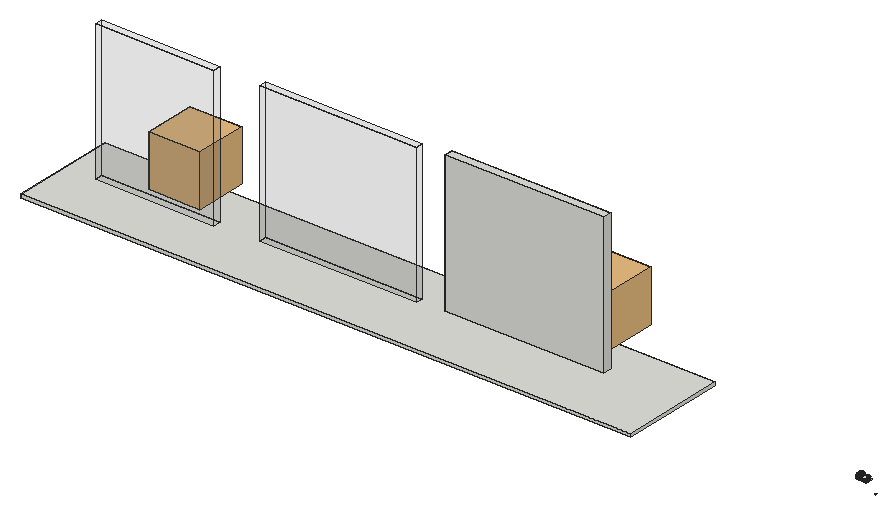
# SketchUp Ruby script. Lengths in inches.
U = 1.inch
M = Sketchup.active_model
def pt(a) = Geom::Point3d.new(a.map { |v| v * U })
def face(e, loops, mat)
  f = e.add_face(loops[0].map { |a| pt(a) })
  loops[1..].each { |l| e.add_face(l.map { |a| pt(a) }).erase! }
  f.material = f.back_material = mat if mat
  f
end
# faces: each face lists its corners as indices into pts; further lists are holes
def faces(e, pts, list, mat = nil) = list.each { |f| face(e, (f[0].is_a?(Array) ? f : [f]).map { |l| l.map { |i| pts[i] } }, mat) }
# xy, xz, yz: faces in a plane at the given z, y or x. An outline is a flat list of corners, or four numbers for a rectangle; further outlines are holes
def ring(l) = l.size == 4 ? [[l[0], l[1]], [l[2], l[1]], [l[2], l[3]], [l[0], l[3]]] : l.each_slice(2).to_a
def flat(e, list, mat, &to3) = list.each { |f| face(e, (f[0].is_a?(Array) ? f : [f]).map { |l| ring(l).map { |u, v| to3.(u, v) } }, mat) }
def xy(e, z, list, mat = nil) = flat(e, list, mat) { |x, y| [x, y, z] }
def xz(e, y, list, mat = nil) = flat(e, list, mat) { |x, z| [x, y, z] }
def yz(e, x, list, mat = nil) = flat(e, list, mat) { |y, z| [x, y, z] }
def lines(e, pts, list) = list.each { |a, b| e.add_line(pt(pts[a]), pt(pts[b])) }
# prism: a flat outline (further loops are holes) pulled along v
def prism(e, loops, v, mat = nil)
  f = face(e, loops, mat); d = Geom::Vector3d.new(v.map { |x| x * U })
  f.pushpull(f.normal.samedirection?(d) ? d.length : -d.length)
end
def box(e, o, s, mat = nil) = prism(e, [[o, [o[0] + s[0], o[1], o[2]], [o[0] + s[0], o[1] + s[1], o[2]], [o[0], o[1] + s[1], o[2]]]], [0, 0, s[2]], mat)
def at(x, y, z, deg = 0) = Geom::Transformation.translation(pt([x, y, z])) * Geom::Transformation.rotation(ORIGIN, Z_AXIS, deg.degrees)
def axes(o, x, y, z) = Geom::Transformation.new([*x, 0, *y, 0, *z, 0, *pt(o).to_a, 1])
def part(name) = M.definitions.add(name)
# library, detail: a bought-in or finely detailed component or shape, given as its bounding box
def library(name, o, s) = part(name).tap { |d| box(d.entities, o, s) }
def detail(e, o, s) = box(e.add_group.entities, o, s)
def put(e, d, t, mat = nil) = e.add_instance(d, t).tap { |i| i.material = mat if mat }
def group(e, t, mat = nil) = e.add_group.tap { |g| g.transformation = t; g.material = mat if mat }.entities
root = M.entities
M.materials.add("GLASS").color = [114, 114, 114]
M.materials["GLASS"].alpha = 0.1
M.materials.add("[Translucent Glass Blue]").color = [100, 149, 237]
M.materials["[Translucent Glass Blue]"].alpha = 0.5
M.materials.add("clear glass").color = [88, 88, 88]
M.materials["clear glass"].alpha = 0.1
c1 = library("sphere",[0,0,0],[319675.55,319675.55,318880.54])
c2 = library("Two-panel window",[0,0,0],[4.33,55.51,41.34])
c3 = library("porta 4",[0.2,-5.42,1.33],[46.55,4.72,83.21])
c4 = library("Group\#52",[0,0,0],[87,177,5.6875])
c5 = part("Group\#55")
box(c5.entities,[0,0,0],[3,19.5,4.5])
c6 = part("Group\#56")
put(c6.entities,c5,at(43.5,84,0))
put(c6.entities,c5,at(61.5,84,0))
put(c6.entities,c5,at(52.5,84,0))
g1 = group(c6.entities,at(0,0,0))
xy(g1,0,[[0,0,0,100.5,43.5,100.5,43.5,87,13.5,87,13.5,0],[94.5,0,94.5,87,46.5,87,46.5,100.5,108,100.5,108,0],[43.5,87,46.5,100.5]])
xy(g1,3,[[0,0,13.5,0,13.5,87,94.5,87,94.5,0,108,0,108,100.5,0,100.5]])
xz(g1,0,[[0,0,13.5,3],[94.5,0,108,3]])
xz(g1,87,[[13.5,0,94.5,3]])
xz(g1,100.5,[[0,0,108,3]])
yz(g1,0,[[0,0,100.5,3]])
yz(g1,13.5,[[0,0,87,3]])
yz(g1,94.5,[[0,0,87,3]])
yz(g1,108,[[0,0,100.5,3]])
p = [[43.5,103.5,0],[46.5,103.5,0],[46.5,84,0],[43.5,84,0],[46.5,87,0],[46.5,100.5,0],
  [43.5,87,0],[43.5,100.5,0]]
lines(g1,p,[[0,1],[2,3],[4,2],[1,5],[3,6],[7,0]])
c7 = library("Group\#33",[0.125,0,0],[4,104,82])
c8 = library("Group\#12",[0,0,0],[11.99,11.97,97.4375])
c9 = library("Group\#11",[0,0,0],[11.99,11.97,97.4375])
c10 = part("Group\#9")
box(c10.entities,[0,0,0],[3,7.87,6])
c11 = library("Group\#10",[0,0,-7.36],[174.08,42.24,224.92])
c12 = part("Difference")
prism(c12.entities,[[[36,15,0],[36,159,0],[0,159,0],[0,462,0],[12,462,0],[12,552,0],[411,552,0],[411,594,0],[774,594,0],[774,27,0],[420,27,0],[420,0,0],[189,0,0],[189,15,0]],[[102.02,387,0],[102.02,208.5,0],[286.5,208.5,0],[286.5,387,0]]],[0,0,6])
c13 = part("Difference\#2")
xy(c13.entities,0,[[177,0,177,15,24,15,24,213,90,213,90,217.5,99,217.5,99,204,33,204,33,24,186,24,186,9,270,9,270,48,274.5,48,274.5,90,270,90,270,198,313.5,198,313.5,258.96,322.5,258.96,322.5,189,279,189,279,99,283.5,99,283.5,39,279,39,279,0],[90,256.5,90,378,24,378,24,462,0,462,0,552,303,552,303,519,307.5,519,307.5,459,303,459,303,435,322.5,435,322.5,305.29,313.5,305.29,313.5,426,294,426,294,468,298.5,468,298.5,510,294,510,294,543,9,543,9,471,33,471,33,387,99,387,99,256.5]])
xy(c13.entities,35.9375,[[24,378,78.91,378,78.91,387,33,387,33,435,24,435]])
xy(c13.entities,36,[[205.5,0,247.5,9],[24,15,81,15,81,24,33,24,33,72,24,72],[144,15,168,24],[90,288,99,359.98],[180,543,204,552],
  [237,543,279,552]])
xy(c13.entities,72,[[237,543,279,552]])
xy(c13.entities,82.0625,[[313.5,258.96,322.5,305.29]])
xy(c13.entities,83.9375,[[24,378,24,435,33,435,33,387,78.91,387,78.91,378]])
xy(c13.entities,84,[[205.5,0,247.5,9],[24,15,24,72,33,72,33,24,81,24,81,15],[144,15,168,24],[90,217.5,99,256.5],[90,288,99,359.98],
  [180,543,204,552]])
xy(c13.entities,120,[[[177,0,279,0,279,39,283.5,39,283.5,99,279,99,279,189,322.5,189,322.5,435,303,435,303,459,307.5,459,307.5,519,303,519,303,552,0,552,0,462,24,462,24,378,90,378,90,213,24,213,24,15,177,15],[186,9,186,24,33,24,33,204,99,204,99,387,33,387,33,471,9,471,9,543,294,543,294,510,298.5,510,298.5,468,294,468,294,426,313.5,426,313.5,198,270,198,270,90,274.5,90,274.5,48,270,48,270,9]]])
xz(c13.entities,0,[[[177,0,279,120],[205.5,36,247.5,84]]])
xz(c13.entities,9,[[[186,0,270,120],[205.5,36,247.5,84]]])
xz(c13.entities,15,[[[24,0,177,0,177,120,24,120,24,84,81,84,81,36,24,36],[144,36,168,84]]])
xz(c13.entities,24,[[[33,0,33,36,81,36,81,84,33,84,33,120,186,120,186,0],[144,36,168,84]]])
xz(c13.entities,39,[[279,0,283.5,120]])
xz(c13.entities,48,[[270,0,274.5,120]])
xz(c13.entities,72,[[24,36,33,84]])
xz(c13.entities,90,[[270,0,274.5,120]])
xz(c13.entities,99,[[279,0,283.5,120]])
xz(c13.entities,189,[[279,0,322.5,120]])
xz(c13.entities,198,[[270,0,313.5,120]])
xz(c13.entities,204,[[33,0,99,120]])
xz(c13.entities,213,[[24,0,90,120]])
xz(c13.entities,217.5,[[90,0,99,84]])
xz(c13.entities,256.5,[[90,0,99,84]])
xz(c13.entities,258.96,[[313.5,0,322.5,82.0625]])
xz(c13.entities,288,[[90,36,99,84]])
xz(c13.entities,305.29,[[313.5,0,322.5,82.0625]])
xz(c13.entities,359.98,[[90,36,99,84]])
xz(c13.entities,378,[[24,0,90,0,90,120,24,120,24,83.9375,78.91,83.9375,78.91,35.9375,24,35.9375]])
xz(c13.entities,387,[[33,0,33,35.9375,78.91,35.9375,78.91,83.9375,33,83.9375,33,120,99,120,99,0]])
xz(c13.entities,426,[[294,0,313.5,120]])
xz(c13.entities,435,[[303,0,322.5,120],[24,35.9375,33,83.9375]])
xz(c13.entities,459,[[303,0,307.5,120]])
xz(c13.entities,462,[[0,0,24,120]])
xz(c13.entities,468,[[294,0,298.5,120]])
xz(c13.entities,471,[[9,0,33,120]])
xz(c13.entities,510,[[294,0,298.5,120]])
xz(c13.entities,519,[[303,0,307.5,120]])
xz(c13.entities,543,[[[9,0,294,120],[237,36,279,72],[180,36,204,84]]])
xz(c13.entities,552,[[[0,0,303,120],[237,36,279,72],[180,36,204,84]]])
yz(c13.entities,0,[[462,0,552,120]])
yz(c13.entities,9,[[471,0,543,120]])
yz(c13.entities,24,[[15,0,15,36,72,36,72,84,15,84,15,120,213,120,213,0],[378,0,378,35.9375,435,35.9375,435,83.9375,378,83.9375,378,120,462,120,462,0]])
yz(c13.entities,33,[[24,0,204,0,204,120,24,120,24,84,72,84,72,36,24,36],[387,0,471,0,471,120,387,120,387,83.9375,435,83.9375,435,35.9375,387,35.9375]])
yz(c13.entities,78.91,[[378,35.9375,387,83.9375]])
yz(c13.entities,81,[[15,36,24,84]])
yz(c13.entities,90,[[[213,0,213,120,378,120,378,0,256.5,0,256.5,84,217.5,84,217.5,0],[288,36,359.98,84]]])
yz(c13.entities,99,[[[204,0,217.5,0,217.5,84,256.5,84,256.5,0,387,0,387,120,204,120],[288,36,359.98,84]]])
yz(c13.entities,144,[[15,36,24,84]])
yz(c13.entities,168,[[15,36,24,84]])
yz(c13.entities,177,[[0,0,15,120]])
yz(c13.entities,180,[[543,36,552,84]])
yz(c13.entities,186,[[9,0,24,120]])
yz(c13.entities,204,[[543,36,552,84]])
yz(c13.entities,205.5,[[0,36,9,84]])
yz(c13.entities,237,[[543,36,552,72]])
yz(c13.entities,247.5,[[0,36,9,84]])
yz(c13.entities,270,[[9,0,48,120],[90,0,198,120]])
yz(c13.entities,274.5,[[48,0,90,120]])
yz(c13.entities,279,[[0,0,39,120],[99,0,189,120],[543,36,552,72]])
yz(c13.entities,283.5,[[39,0,99,120]])
yz(c13.entities,294,[[426,0,468,120],[510,0,543,120]])
yz(c13.entities,298.5,[[468,0,510,120]])
yz(c13.entities,303,[[435,0,459,120],[519,0,552,120]])
yz(c13.entities,307.5,[[459,0,519,120]])
yz(c13.entities,313.5,[[198,0,198,120,426,120,426,0,305.29,0,305.29,82.0625,258.96,82.0625,258.96,0]])
yz(c13.entities,322.5,[[189,0,258.96,0,258.96,82.0625,305.29,82.0625,305.29,0,435,0,435,120,189,120]])
c14 = part("Group140\#1")
box(c14.entities,[66627.7,5273.03,126],[1.73,0.47,42.84])
box(c14.entities,[66627.7,5365.51,126],[1.73,0.47,42.84])
box(c14.entities,[66627.7,5457.99,126],[1.73,0.47,42.84])
box(c14.entities,[66627.7,5550.46,126],[1.73,0.48,42.84])
box(c14.entities,[66627.7,5642.94,126],[1.73,0.48,42.84])
c15 = part("Group149\#1")
box(c15.entities,[66628.33,5734.79,126],[0.47,1.74,42.84])
c16 = part("Group150\#1")
box(c16.entities,[66542.5625,5734.79,126],[0.48,1.74,42.84])
box(c16.entities,[66456.8,5734.79,126],[0.47,1.74,42.84])
box(c16.entities,[66371.03,5734.79,126],[0.48,1.74,42.84])
c17 = part("Group151\#1")
box(c17.entities,[66285.27,5734.79,168.84],[343.53,1.74,0.47])
c18 = part("Group145\#1")
box(c18.entities,[66558.33,5179.92,126],[0.47,1.73,42.84])
c19 = part("Group139\#1")
box(c19.entities,[66627.7,5735.42,126],[1.73,0.48,42.84])
c20 = part("Group149\#2")
box(c20.entities,[66285.27,5734.79,126],[0.47,1.74,42.84])
c21 = part("Group154\#1")
box(c21.entities,[66284.64,5735.42,126],[1.73,0.48,42.84])
c22 = part("Group152\#1")
box(c22.entities,[66285.5,5734.79,134.39],[343.07,1.74,0.36])
box(c22.entities,[66285.5,5734.79,142.96],[343.07,1.74,0.35])
box(c22.entities,[66285.5,5734.79,151.53],[343.07,1.74,0.35])
box(c22.entities,[66285.5,5734.79,160.09],[343.07,1.74,0.36])
c23 = part("Difference\#3")
xy(c23.entities,0,[[0,0,0,130.5,189,130.5,189,70.4,180,70.4,180,121.5,9,121.5,9,9,180,9,180,22.4,189,22.4,189,0]])
xy(c23.entities,36,[[57,0,138,9]])
xy(c23.entities,84,[[57,0,138,9],[180,22.4,189,70.4]])
xy(c23.entities,120,[[[0,0,189,130.5],[9,9,180,121.5]]])
xz(c23.entities,0,[[[0,0,189,120],[57,36,138,84]]])
xz(c23.entities,9,[[[9,0,180,120],[57,36,138,84]]])
xz(c23.entities,22.4,[[180,0,189,84]])
xz(c23.entities,70.4,[[180,0,189,84]])
xz(c23.entities,121.5,[[9,0,180,120]])
xz(c23.entities,130.5,[[0,0,189,120]])
yz(c23.entities,0,[[0,0,130.5,120]])
yz(c23.entities,9,[[9,0,121.5,120]])
yz(c23.entities,57,[[0,36,9,84]])
yz(c23.entities,138,[[0,36,9,84]])
yz(c23.entities,180,[[9,0,9,120,121.5,120,121.5,0,70.4,0,70.4,84,22.4,84,22.4,0]])
yz(c23.entities,189,[[0,0,22.4,0,22.4,84,70.4,84,70.4,0,130.5,0,130.5,120,0,120]])
c24 = library("Group\#53",[0,0,0],[63,171,4.5])
c25 = part("Group161\#1")
box(c25.entities,[66179.57,5691.79,134.39],[105.93,1.74,0.36])
box(c25.entities,[66179.57,5691.79,142.96],[105.93,1.74,0.35])
box(c25.entities,[66179.57,5691.79,151.53],[105.93,1.74,0.35])
box(c25.entities,[66179.57,5691.79,160.09],[105.93,1.74,0.36])
c26 = part("Group158\#1")
box(c26.entities,[66285.27,5691.79,126],[0.47,1.74,42.84])
c27 = part("Group156\#2")
box(c27.entities,[66284.64,5692.66,134.39],[1.73,43,0.36])
box(c27.entities,[66284.64,5692.66,142.96],[1.73,43,0.35])
box(c27.entities,[66284.64,5692.66,151.53],[1.73,43,0.35])
box(c27.entities,[66284.64,5692.66,160.09],[1.73,43,0.36])
c28 = part("Group156\#1")
box(c28.entities,[66284.64,5692.42,168.84],[1.73,43.48,0.47])
c29 = part("Group158\#2")
box(c29.entities,[66179.33,5691.79,126],[0.47,1.74,42.84])
c30 = part("Group154\#2")
box(c30.entities,[66284.64,5692.42,126],[1.73,0.48,42.84])
c31 = part("Group160\#1")
box(c31.entities,[66179.33,5691.79,168.84],[106.41,1.74,0.47])
c32 = part("Group159\#1")
box(c32.entities,[66232.3,5691.79,126],[0.47,1.74,42.84])
c33 = library("Group\#20",[1.1875,0,0],[59.6875,59.6875,48])
c34 = part("Group\#25")
xy(c34.entities,0,[[0,0,50.69,0,50.69,0.34,0.34,0.34,0.34,51.19,0,51.19],[0.53,0.53,50.69,0.53,50.69,0.875,0.875,0.875,0.875,51.19,0.53,51.19]])
xy(c34.entities,41.65,[[0.34,0.34,50.69,0.34,50.69,0.53,0.53,0.53,0.53,51.19,0.34,51.19]])
xz(c34.entities,0.34,[[0.34,0,50.69,41.65]])
xz(c34.entities,0.53,[[0.53,0,50.69,41.65]])
xz(c34.entities,51.19,[[0.34,0,0.53,41.65]])
yz(c34.entities,0.34,[[0.34,0,51.19,41.65]])
yz(c34.entities,0.53,[[0.53,0,51.19,41.65]])
yz(c34.entities,50.69,[[0.34,0,0.53,41.65]])
c35 = part("Group\#24")
xy(c35.entities,0,[[0,0,0,54.6875,1.5625,54.6875,1.5625,1.5625,54.1875,1.5625,54.1875,0]])
xy(c35.entities,2.0625,[[0,0,52.125,0,52.125,0.32,0.32,0.32,0.32,52.625,0,52.625],[1.2,1.2,52.125,1.2,52.125,1.5625,1.5625,1.5625,1.5625,52.625,1.2,52.625]])
xy(c35.entities,3.18,[[0.32,0.32,51.01,0.32,51.01,1.2,1.2,1.2,1.2,51.51,0.32,51.51]])
xy(c35.entities,44.82,[[0.32,0.32,0.32,51.51,1.2,51.51,1.2,1.2,51.01,1.2,51.01,0.32]])
xy(c35.entities,45.9375,[[0,0,0,52.625,0.32,52.625,0.32,0.32,52.125,0.32,52.125,0],[1.2,1.2,1.2,52.625,1.5625,52.625,1.5625,1.5625,52.125,1.5625,52.125,1.2]])
xy(c35.entities,48,[[0,0,54.1875,0,54.1875,1.5625,1.5625,1.5625,1.5625,54.6875,0,54.6875]])
xz(c35.entities,0,[[0,0,54.1875,0,54.1875,48,0,48,0,45.9375,52.125,45.9375,52.125,2.0625,0,2.0625]])
xz(c35.entities,0.32,[[0.32,2.0625,52.125,2.0625,52.125,45.9375,0.32,45.9375,0.32,44.82,51.01,44.82,51.01,3.18,0.32,3.18]])
xz(c35.entities,1.2,[[1.2,2.0625,1.2,3.18,51.01,3.18,51.01,44.82,1.2,44.82,1.2,45.9375,52.125,45.9375,52.125,2.0625]])
xz(c35.entities,1.5625,[[1.5625,0,1.5625,2.0625,52.125,2.0625,52.125,45.9375,1.5625,45.9375,1.5625,48,54.1875,48,54.1875,0]])
xz(c35.entities,51.51,[[0.32,3.18,1.2,44.82]])
xz(c35.entities,52.625,[[0,2.0625,0.32,45.9375],[1.2,2.0625,1.5625,45.9375]])
xz(c35.entities,54.6875,[[0,0,1.5625,48]])
yz(c35.entities,0,[[0,0,0,2.0625,52.625,2.0625,52.625,45.9375,0,45.9375,0,48,54.6875,48,54.6875,0]])
yz(c35.entities,0.32,[[0.32,2.0625,0.32,3.18,51.51,3.18,51.51,44.82,0.32,44.82,0.32,45.9375,52.625,45.9375,52.625,2.0625]])
yz(c35.entities,1.2,[[1.2,2.0625,52.625,2.0625,52.625,45.9375,1.2,45.9375,1.2,44.82,51.51,44.82,51.51,3.18,1.2,3.18]])
yz(c35.entities,1.5625,[[1.5625,0,54.6875,0,54.6875,48,1.5625,48,1.5625,45.9375,52.625,45.9375,52.625,2.0625,1.5625,2.0625]])
yz(c35.entities,51.01,[[0.32,3.18,1.2,44.82]])
yz(c35.entities,52.125,[[0,2.0625,0.32,45.9375],[1.2,2.0625,1.5625,45.9375]])
yz(c35.entities,54.1875,[[0,0,1.5625,48]])
c36 = part("Group141\#1")
box(c36.entities,[66627.7,5180.55,168.84],[1.73,555.35,0.47])
c37 = part("Group142\#1")
box(c37.entities,[66627.7,5180.78,134.39],[1.73,554.88,0.36])
box(c37.entities,[66627.7,5180.78,142.96],[1.73,554.88,0.35])
box(c37.entities,[66627.7,5180.78,151.53],[1.73,554.88,0.35])
box(c37.entities,[66627.7,5180.78,160.09],[1.73,554.88,0.36])
c38 = part("Group138\#1")
box(c38.entities,[66627.7,5180.55,126],[1.73,0.47,42.84])
c39 = part("Group144\#2")
box(c39.entities,[66628.33,5179.92,126],[0.47,1.73,42.84])
c40 = part("Group146\#1")
box(c40.entities,[66488.33,5179.92,168.84],[140.47,1.73,0.47])
c41 = part("Group147\#1")
box(c41.entities,[66488.57,5179.92,134.39],[140,1.73,0.36])
box(c41.entities,[66488.57,5179.92,142.96],[140,1.73,0.35])
box(c41.entities,[66488.57,5179.92,151.53],[140,1.73,0.35])
box(c41.entities,[66488.57,5179.92,160.09],[140,1.73,0.36])
c42 = part("Group144\#1")
box(c42.entities,[66488.33,5179.92,126],[0.47,1.73,42.84])
prism(root,[[[65574.81,5459.59,258],[65877.81,5459.59,258],[65877.81,5426.59,258],[65882.31,5426.59,258],[65882.31,5342.59,258],[65897.31,5342.59,258],[65897.31,5324.59,258],[66012.79,5324.59,258],[66012.79,5066.59,258],[65853.81,5066.59,258],[65853.81,5006.59,258],[65858.31,5006.59,258],[65858.31,4916.59,258],[65895.75,4916.59,258],[65895.75,4880.59,258],[65804.81,4880.59,258],[65804.81,4865.59,258],[65691.31,4865.59,258],[65691.31,4880.59,258],[65598.81,4880.59,258],[65598.81,5066.59,258],[65562.81,5066.59,258],[65562.81,5360.42,258],[65574.81,5360.42,258]],[[65576.1875,5347.05,258],[65576.1875,5079.97,258],[65612.1875,5079.97,258],[65612.1875,4893.97,258],[65704.6875,4893.97,258],[65704.6875,4878.97,258],[65791.43,4878.97,258],[65791.43,4893.97,258],[65882.37,4893.97,258],[65882.37,4903.21,258],[65844.93,4903.21,258],[65844.93,4993.21,258],[65840.43,4993.21,258],[65840.43,5079.97,258],[65999.41,5079.97,258],[65999.41,5311.21,258],[65883.93,5311.21,258],[65883.93,5329.21,258],[65868.93,5329.21,258],[65868.93,5413.21,258],[65864.43,5413.21,258],[65864.43,5446.21,258],[65588.1875,5446.21,258],[65588.1875,5347.05,258]]],[0,0,38.0625])
xy(root,102,[[66327.81,5258.6,66336.81,5315.6]])
xy(root,132,[[65853.81,4880.59,65982.81,4884.84],[65977.96,4884.84,65982.81,4915.03]])
xy(root,168,[[65853.81,4880.59,65982.81,4880.59,65982.81,4915.03,65977.96,4915.03,65977.96,4884.84,65853.81,4884.84]])
xy(root,378,[[65673.79,5167.59,65673.79,5303.59,65673.81,5303.59],[65673.79,5167.59,65673.81,5303.59,65862.79,5303.59,65862.79,5294.59,65858.29,5294.59,65858.29,5167.59,65849.29,5167.59,65849.29,5294.59,65682.81,5294.59,65682.79,5185.59,65796.79,5185.59,65796.79,5215.59,65805.79,5215.59,65805.79,5167.59],[65805.79,5167.59,65805.79,5215.59,65796.79,5215.59,65796.79,5185.59,65682.79,5185.59,65682.81,5294.59,65849.29,5294.59,65849.29,5167.59],[65858.29,5167.59,65862.79,5294.59]])
xy(root,384,[[[65657.41,5151.21,65879.17,5319.97],[65673.79,5167.59,65862.79,5303.59]]])
xy(root,390,[[[65657.41,5151.21,65879.17,5319.97],[65673.79,5167.59,65862.79,5303.59]]])
xy(root,395.9375,[[[65657.41,5151.21,65879.17,5319.97],[65673.79,5167.59,65862.79,5303.59]]])
xy(root,401.9375,[[65657.41,5151.21,65879.17,5319.97]])
xz(root,4880.59,[[65853.81,132,65982.81,168]])
xz(root,4884.84,[[65853.81,132,65977.96,168]])
xz(root,4915.03,[[65977.96,132,65982.81,168]])
xz(root,5151.21,[[65657.41,384,65879.17,390],[65657.41,395.9375,65879.17,401.9375]])
xz(root,5167.59,[[65673.79,378,65862.79,384],[65673.79,384,65862.79,390],[65673.79,390,65862.79,395.9375]])
xz(root,5303.59,[[65673.79,378,65862.79,384],[65673.79,384,65862.79,390],[65673.79,390,65862.79,395.9375]])
xz(root,5315.6,[[66327.81,54,66336.81,102]])
xz(root,5319.97,[[65657.41,384,65879.17,390],[65657.41,395.9375,65879.17,401.9375]])
yz(root,65657.41,[[5151.21,384,5319.97,390],[5151.21,395.9375,5319.97,401.9375]])
yz(root,65673.79,[[5167.59,378,5303.59,384],[5167.59,384,5303.59,390],[5167.59,390,5303.59,395.9375]])
yz(root,65853.81,[[4880.59,132,4884.84,168]])
yz(root,65862.79,[[5167.59,378,5303.59,384],[5167.59,384,5303.59,390],[5167.59,390,5303.59,395.9375]])
yz(root,65879.17,[[5151.21,384,5319.97,390],[5151.21,395.9375,5319.97,401.9375]])
yz(root,65977.96,[[4884.84,132,4915.03,168]])
yz(root,65982.81,[[4880.59,132,4915.03,168]])
yz(root,66327.81,[[[5196.39,6,5196.39,90,5149.84,90,5149.84,126,5423.6,126,5423.6,6],[5257.47,52.625,5315.6,102]]])
p = [[66336.81,5258.6,54],[66336.81,5315.6,54],[66336.81,5258.6,102],[66240.59,4903.1,6],[66240.59,4907.6,6],[66177.59,4903.1,6],
  [65598.81,5093.6,6],[65598.81,4895.6,6],[65838.81,4878.03,6],[65838.81,4877.09,6],[66083.31,4904.6,6],[66096.81,4904.6,6],
  [66336.81,4907.6,6],[66336.81,5432.6,6],[65829.81,4878.03,6],[65838.37,4878.03,6],[65751.81,4895.6,6],[65751.81,4880.59,6],
  [66066.81,5432.6,6],[65973.81,5432.6,6],[65574.81,5432.6,6],[65574.81,5342.6,6],[65973.81,5456.6,6],[66066.81,5456.6,6],
  [65988.81,4904.6,6],[66002.31,4904.6,6],[65829.81,4880.59,6],[66096.81,4904.6,6.75],[65982.81,4907.6,6],[65988.81,4907.6,6],
  [65598.81,5342.6,6],[65849.29,5294.59,258],[65849.29,5206.59,258],[65673.79,5167.59,258],[65673.79,5294.59,258],[65916.81,4880.53,6],
  [65916.81,4880.59,6],[65809.6,5167.59,258],[65849.29,5167.59,258],[65916.81,4878.03,6],[65907.81,4877.09,6],[65907.81,4878.03,6],
  [66177.59,4907.6,6],[66083.31,4907.6,6],[66002.31,4907.6,6],[65982.81,4880.53,6],[65598.81,5258.6,6],[65664.81,5258.6,6],
  [65664.81,5093.6,6]]
lines(root,p,[[0,1],[2,0],[3,4],[5,3],[6,7],[8,9],[10,11],[12,13],[14,15],[15,8],[16,17],[13,18],
  [19,20],[20,21],[22,19],[4,12],[18,23],[24,25],[17,26],[11,27],[28,29],[21,30],[31,32],[33,34],
  [34,31],[35,36],[23,22],[37,33],[32,38],[38,37],[39,35],[9,40],[40,41],[27,42],[43,10],[25,44],
  [36,45],[30,46],[47,48],[29,24],[45,28],[41,39],[46,47],[26,14],[35,45],[7,16],[44,43],[42,5],
  [48,6]])
detail(root,[66171.59,4897.16,168.83],[75,10.44,13.82])
put(root,c1,axes([6086.83,5705.64,280.5],[0.01346,0,0],[0,0.01346,0],[0,0,0.01346]))
put(root,c1,axes([38489.33,7812.39,280.5],[0.01346,0,0],[0,0.01346,0],[0,0,0.01346]))
put(root,c2,axes([65742.81,4897.93,42],[0,1,0],[-0.43234,0,0],[0,0,1.16114]))
put(root,c2,axes([65822.31,4882.93,168],[0,1,0],[-0.7566,0,0],[0,0,1.16114]))
put(root,c2,axes([66041.28,5447.7,42],[0,1.53909,0],[-0.75615,0,0],[0,0,1.16114]))
put(root,c2,axes([66144.81,4909.93,42],[0,1,0],[-0.43234,0,0],[0,0,1.16114]))
put(root,c2,axes([66180.81,5425.53,42],[0,1,0],[-0.43234,0,0],[0,0,1.16114]))
put(root,c2,axes([65946.81,5421.43,42],[0,1.53909,0],[-0.75615,0,0],[0,0,1.16114]))
put(root,c2,axes([66123.78,5423.7,42],[0,1.53909,0],[-0.75615,0,0],[0,0,1.16114]))
put(root,c2,axes([65778.81,5426.03,42],[0,1,0],[-0.43234,0,0],[0,0,1.16114]))
put(root,c2,axes([65742.81,4897.93,168],[0,1,0],[-0.43234,0,0],[0,0,1.16114]))
put(root,c3,axes([65863.49,5238.61,256.67],[0,-1.04,0],[1,0,0],[0,0,1]))
put(root,c2,axes([65820.81,4881.76,42],[0,1.53909,0],[-0.64851,0,0],[0,0,1.16114]))
put(root,c3,at(65899.16,5185.93,129.4,-90))
put(root,c3,at(66340.6,5196.59,6,-90))
put(root,c2,axes([65778.81,5426.03,168],[0,1,0],[-0.43234,0,0],[0,0,1.16114]))
put(root,c2,axes([65853.81,5421.43,42],[0,1.53909,0],[-0.75615,0,0],[0,0,1.16114]))
put(root,c2,axes([65853.81,5423.12,168],[0,1.53909,0],[-0.75615,0,0],[0,0,1.16114]))
put(root,c3,axes([65666.19,5140.34,131.49],[0,-1,0],[0.35,0,0],[0,0,1]))
g2 = group(root,at(0,0,0))
box(g2,[0,0,0],[50758.8125,8802,280.5])
g3 = group(root,at(2625.375,4519.88,280.5),"GLASS")
box(g3,[0,0,0],[9888.0625,704.75,11609.4375],"GLASS")
g4 = group(root,at(16056.5,4790.28,280.5))
box(g4,[0,0,0],[13076.125,643.8125,11609.4375],"clear glass")
g5 = group(root,at(31168.76,5181.86,280.5))
g6 = group(g5,at(0,0,0))
box(g6,[0,0,0],[13237.875,743.9375,11609.4375])
g7 = group(root,at(67840.39,4008.42,0))
prism(g7,[[[107,0,0],[94,0,0],[94,53.5,0],[13,53.5,0],[13,0,0],[0,0,0],[0,66.5,0],[107,66.5,0]]],[0,0,7.125])
p = [[89.5,0,0],[94,0,0]]
lines(g7,p,[[0,1]])
g8 = group(root,at(65574.81,4880.59,0))
prism(g8,[[[24,15,0],[24,213,0],[90,213,0],[90,378,0],[24,378,0],[24,462,0],[0,462,0],[0,552,0],[399,552,0],[399,576,0],[492,576,0],[492,552,0],[909.875,552,0],[909.875,27,0],[408,27,0],[408,0,0],[177,0,0],[177,15,0]]],[0,0,6])
put(root,c4,axes([65829.81,4880.53,6],[1,0,0],[0,0,1],[0,-1,0]))
put(root,c6,axes([65717.29,5167.59,258],[1,0,0],[0,0,1],[0,-1,0]))
put(root,c7,axes([65666.9,5168.6,42],[0.55,0,0],[0,0.70686,0],[0,0,0.58537]))
put(root,c8,at(66468.82,5081.61,5.5))
put(root,c9,at(66468.81,5258.6,5.5))
g9 = group(root,at(65706.43,5281.51,431.18))
box(g9,[0,-93.875,0],[132,93.875,3])
put(root,c10,axes([65763.81,5230.72,370.13],[1,0,0],[0,0,1],[0,-1,0]))
put(root,c10,axes([65682.81,5230.72,370.13],[1,0,0],[0,0,1],[0,-1,0]))
put(root,c10,axes([65682.81,5294.59,370.13],[1,0,0],[0,0,1],[0,-1,0]))
g10 = group(root,at(65718.08,5269.51,401.9375))
box(g10,[0,-69.875,0],[108.35,69.875,29.25])
put(root,c10,axes([65763.81,5294.59,370.13],[1,0,0],[0,0,1],[0,-1,0]))
g11 = group(root,at(66249.8125,4883.6,90))
prism(g11,[[[0,24,0],[87,24,0],[87,111,0],[111,111,0],[111,0,0],[0,0,0]]],[0,0,8.0625])
put(root,c11,axes([66336.81,5281.23,89.76],[1,0,0],[0,0,1],[0,-1,0]))
put(root,c12,at(65562.81,4880.59,126))
put(root,c13,at(65574.81,4880.59,132))
put(root,c6,axes([65988.81,4907.6,6],[1,0,0],[0,0,1],[0,-1,0]))
put(root,c14,at(-301.76,-269.47,6))
put(root,c15,at(-301.76,-269.47,6))
put(root,c16,at(-301.76,-269.47,6))
put(root,c17,at(-301.76,-269.47,6))
put(root,c18,at(-318.08,-269.43,6.47))
put(root,c19,at(-301.76,-269.47,6))
put(root,c20,at(-301.76,-269.47,6))
put(root,c21,at(-301.76,-269.47,6))
put(root,c22,at(-301.76,-269.47,6))
put(root,c7,axes([66078.88,4911.33,42],[0,0.55,0],[-0.693,0,0],[0,0,0.58537]))
put(root,c23,at(65673.79,5167.59,258))
g12 = group(root,at(65982.81,4915.03,132))
prism(g12,[[[204,-7.4375,0],[204,-7.4375,36],[0,-7.4375,36],[0,-7.4375,0]],[[93,-7.4375,30],[97.5,-7.4375,30],[97.5,-7.4375,12],[93,-7.4375,12]],[[120,-7.4375,30],[120,-7.4375,12],[115.5,-7.4375,12],[115.5,-7.4375,30]],[[25.5,-7.4375,30],[30,-7.4375,30],[30,-7.4375,12],[25.5,-7.4375,12]],[[48,-7.4375,30],[52.5,-7.4375,30],[52.5,-7.4375,12],[48,-7.4375,12]],[[75,-7.4375,12],[70.5,-7.4375,12],[70.5,-7.4375,30],[75,-7.4375,30]],[[142.5,-7.4375,12],[138,-7.4375,12],[138,-7.4375,30],[142.5,-7.4375,30]],[[160.5,-7.4375,12],[160.5,-7.4375,30],[165,-7.4375,30],[165,-7.4375,12]],[[183,-7.4375,12],[183,-7.4375,30],[187.5,-7.4375,30],[187.5,-7.4375,12]]],[0,7.4375,0])
g13 = group(root,at(65562.81,4865.59,252))
xy(g13,0,[[[128.5,0,128.5,15,36,15,36,201,0,201,0,494.83,12,494.83,12,594,315,594,315,561,319.5,561,319.5,477,334.5,477,334.5,459,449.98,459,449.98,201,291,201,291,141,295.5,141,295.5,51,332.9375,51,332.9375,15,242,15,242,0],[110.98,302,286.48,429]]])
xy(g13,6,[[[128.5,0,242,0,242,15,332.9375,15,332.9375,51,295.5,51,295.5,141,291,141,291,201,449.98,201,449.98,459,334.5,459,334.5,477,319.5,477,319.5,561,315,561,315,594,12,594,12,494.83,0,494.83,0,201,36,201,36,15,128.5,15],[110.98,302,286.48,429]]])
xz(g13,0,[[128.5,0,242,6]])
xz(g13,15,[[36,0,128.5,6],[242,0,332.9375,6]])
xz(g13,51,[[295.5,0,332.9375,6]])
xz(g13,141,[[291,0,295.5,6]])
xz(g13,201,[[0,0,36,6],[291,0,449.98,6]])
xz(g13,302,[[110.98,0,286.48,6]])
xz(g13,429,[[110.98,0,286.48,6]])
xz(g13,459,[[334.5,0,449.98,6]])
xz(g13,477,[[319.5,0,334.5,6]])
xz(g13,494.83,[[0,0,12,6]])
xz(g13,561,[[315,0,319.5,6]])
xz(g13,594,[[12,0,315,6]])
yz(g13,0,[[201,0,494.83,6]])
yz(g13,12,[[494.83,0,594,6]])
yz(g13,36,[[15,0,201,6]])
yz(g13,110.98,[[302,0,429,6]])
yz(g13,128.5,[[0,0,15,6]])
yz(g13,242,[[0,0,15,6]])
yz(g13,286.48,[[302,0,429,6]])
yz(g13,291,[[141,0,201,6]])
yz(g13,295.5,[[51,0,141,6]])
yz(g13,315,[[561,0,594,6]])
yz(g13,319.5,[[477,0,561,6]])
yz(g13,332.9375,[[15,0,51,6]])
yz(g13,334.5,[[459,0,477,6]])
yz(g13,449.98,[[201,0,459,6]])
put(root,c7,axes([65813.18,5172.02,293.85],[0,0.55,0],[-0.85239,0,0],[0,0,0.58537]))
g14 = group(root,at(66116.76,4883.6,90))
box(g14,[0,0,0],[32.48,24,6])
g15 = group(root,at(65901.54,4856.59,89.5))
prism(g15,[[[15.64,0,0],[15.375,24,0],[81.26,24,0],[81.26,51,0],[105.26,51,0],[105.26,0,0]]],[0,0,6])
g16 = group(root,at(65712.4,4871.6,90))
box(g16,[0,0,0],[36.09,24,6])
g17 = group(root,at(65778.81,4856.59,90))
box(g17,[0,0,0],[48,24,6])
g18 = group(root,at(65730.81,5432.6,90))
box(g18,[0,0,0],[147,24,6])
g19 = group(root,at(65574.81,4871.6,90))
prism(g19,[[[0,105,0],[24,105,0],[24,24,0],[105,24,0],[105,0,0],[0,0,0]]],[0,0,6])
put(root,c24,axes([66177.59,4907.6,6],[1,0,0],[0,0,1],[0,-1,0]))
put(root,c25,at(-301.76,-269.47,6))
put(root,c26,at(-301.76,-269.47,6))
put(root,c27,at(-301.76,-269.47,6))
put(root,c28,at(-301.76,-269.47,6))
put(root,c29,at(-301.76,-269.47,6))
put(root,c30,at(-301.76,-269.47,6))
put(root,c31,at(-301.76,-269.47,6))
put(root,c32,at(-301.76,-269.47,6))
put(root,c33,at(66272.62,4910.91,42))
g20 = group(root,at(66274.39,4911.33,43.77),"[Translucent Glass Blue]")
prism(g20,[[[57.51,57.5,0],[57.5,0,0],[0,0,0],[0,0.08,0],[57.42,0.08,0],[57.43,57.5,0]]],[0,0,44.46])
g21 = group(root,at(65925.81,4884.03,42))
xy(g21,0,[[0,0,0,0.625,52.9375,0.625,52.9375,23.57,53.5625,23.57,53.5625,0]])
xy(g21,0.875,[[0.875,0,53.5625,0,53.5625,22.69,53.34,22.69,53.34,0.23,0.875,0.23],[0.875,0.41,53.15,0.41,53.15,22.69,52.9375,22.69,52.9375,0.625,0.875,0.625]])
xy(g21,1.16,[[1.16,0.23,53.34,0.23,53.34,22.4,53.15,22.4,53.15,0.41,1.16,0.41]])
xy(g21,46.84,[[1.16,0.23,1.16,0.41,53.15,0.41,53.15,22.4,53.34,22.4,53.34,0.23]])
xy(g21,47.125,[[0.875,0,0.875,0.23,53.34,0.23,53.34,22.69,53.5625,22.69,53.5625,0],[0.875,0.41,0.875,0.625,52.9375,0.625,52.9375,22.69,53.15,22.69,53.15,0.41]])
xy(g21,48,[[0,0,53.5625,0,53.5625,23.57,52.9375,23.57,52.9375,0.625,0,0.625]])
xz(g21,0,[[0,0,53.5625,0,53.5625,0.875,0.875,0.875,0.875,47.125,53.5625,47.125,53.5625,48,0,48]])
xz(g21,0.23,[[0.875,0.875,53.34,0.875,53.34,1.16,1.16,1.16,1.16,46.84,53.34,46.84,53.34,47.125,0.875,47.125]])
xz(g21,0.41,[[0.875,0.875,0.875,47.125,53.15,47.125,53.15,46.84,1.16,46.84,1.16,1.16,53.15,1.16,53.15,0.875]])
xz(g21,0.625,[[0,0,0,48,52.9375,48,52.9375,47.125,0.875,47.125,0.875,0.875,52.9375,0.875,52.9375,0]])
xz(g21,22.4,[[53.15,1.16,53.34,46.84]])
xz(g21,22.69,[[52.9375,0.875,53.15,47.125],[53.34,0.875,53.5625,47.125]])
xz(g21,23.57,[[52.9375,0,53.5625,48]])
yz(g21,0,[[0,0,0.625,48]])
yz(g21,0.875,[[0,0.875,0.23,47.125],[0.41,0.875,0.625,47.125]])
yz(g21,1.16,[[0.23,1.16,0.41,46.84]])
yz(g21,52.9375,[[0.625,0,0.625,0.875,22.69,0.875,22.69,47.125,0.625,47.125,0.625,48,23.57,48,23.57,0]])
yz(g21,53.15,[[0.41,0.875,0.41,1.16,22.4,1.16,22.4,46.84,0.41,46.84,0.41,47.125,22.69,47.125,22.69,0.875]])
yz(g21,53.34,[[0.23,0.875,22.69,0.875,22.69,47.125,0.23,47.125,0.23,46.84,22.4,46.84,22.4,1.16,0.23,1.16]])
yz(g21,53.5625,[[0,0,23.57,0,23.57,48,0,48,0,47.125,22.69,47.125,22.69,0.875,0,0.875]])
put(root,c34,at(65601.94,4898.23,45.18),"[Translucent Glass Blue]")
put(root,c35,at(65601.62,4897.91,42))
put(root,c35,at(65601.62,5260.91,42))
g22 = group(root,at(65926.97,4884.25,43.16),"[Translucent Glass Blue]")
xy(g22,0,[[0,0,52.17,0,52.17,22.18,52.09,22.18,52.11,0.07,0,0.07],[0,0.12,52.05,0.12,52.03,22.18,51.99,22.18,51.99,0.1875,0,0.1875]])
xy(g22,45.67,[[0,0.07,52.11,0.07,52.09,22.18,52.03,22.18,52.05,0.12,0,0.12]])
xz(g22,0.07,[[0,0,52.11,45.67]])
xz(g22,0.12,[[0,0,52.05,45.67]])
xz(g22,22.18,[[52.03,0,52.09,45.67]])
yz(g22,0,[[0.07,0,0.12,45.67]])
p = [[52.03,22.18,0],[52.05,0.12,0],[52.05,0.12,45.67],[52.03,22.18,45.67],[52.11,0.07,0],[52.09,22.18,0],
  [52.09,22.18,45.67],[52.11,0.07,45.67]]
faces(g22,p,[[0,1,2,3],[4,5,6,7]])
put(root,c34,at(65601.94,5261.23,45.18),"[Translucent Glass Blue]")
put(root,c34,at(65601.94,4898.23,171.18),"[Translucent Glass Blue]")
put(root,c35,at(65601.62,4897.91,168))
put(root,c34,at(65601.94,5261.23,171.11),"[Translucent Glass Blue]")
put(root,c35,at(65601.62,5260.91,167.9375))
put(root,c7,axes([65669.24,5167.21,167.85],[0.55,0,0],[0,0.70686,0],[0,0,0.58537]))
g23 = group(root,at(65574.81,4880.59,6))
xy(g23,0,[[177,0,177,15,24,15,24,213,90,213,90,378,24,378,24,462,0,462,0,552,399,552,399,576,492,576,492,552,762,552,762,435,753,435,753,543,483,543,483,567,408,567,408,543,9,543,9,471,33,471,33,387,99,387,99,204,33,204,33,24,186,24,186,9,399,9,399,36,753,36,753,269.25,762,269.25,762,27,408,27,408,0],[753,315.8,762,378],[753,378,762,435]])
xy(g23,36,[[210,0,246,9],[351,0,408,0,408,27,399,27,399,9,351,9],[24,15,81,15,81,24,33,24,33,72,24,72],[144,15,168,24],[432,27,504,36],
  [546,27,570,36],[699,27,762,27,762,90,753,90,753,36,699,36],[90,288,99,359.98],[24,378,81,378,81,387,33,387,33,435,24,435],[180,543,204,552],
  [237,543,279,552],[330,543,372,552],[507,543,549,552],[582,543,606,552],[424.5,567,466.5,576]])
xy(g23,84,[[210,0,246,9],[351,0,351,9,399,9,399,27,408,27,408,0],[24,15,24,72,33,72,33,24,81,24,81,15],[144,15,168,24],[432,27,504,36],
  [546,27,570,36],[699,27,699,36,753,36,753,90,762,90,762,27],[753,269.25,762,315.8],[90,288,99,359.98],[24,378,24,435,33,435,33,387,81,387,81,378],
  [180,543,204,552],[237,543,279,552],[330,543,372,552],[507,543,549,552],[582,543,606,552],
  [424.5,567,466.5,576]])
xy(g23,120,[[177,0,408,0,408,27,762,27,762,269.25,753,269.25,753,36,399,36,399,9,186,9,186,24,33,24,33,204,99,204,99,387,33,387,33,471,9,471,9,543,408,543,408,567,483,567,483,543,753,543,753,269.25,762,269.25,762,552,492,552,492,576,399,576,399,552,0,552,0,462,24,462,24,378,90,378,90,213,24,213,24,15,177,15]])
xz(g23,0,[[[177,0,408,0,408,36,351,36,351,84,408,84,408,120,177,120],[210,36,246,84]]])
xz(g23,9,[[[186,0,186,120,399,120,399,84,351,84,351,36,399,36,399,0],[210,36,246,84]]])
xz(g23,15,[[[24,0,177,0,177,120,24,120,24,84,81,84,81,36,24,36],[144,36,168,84]]])
xz(g23,24,[[[33,0,33,36,81,36,81,84,33,84,33,120,186,120,186,0],[144,36,168,84]]])
xz(g23,27,[[[408,0,762,0,762,36,699,36,699,84,762,84,762,120,408,120,408,84,399,84,399,36,408,36],[432,36,504,84],[546,36,570,84]]])
xz(g23,36,[[[399,0,399,120,753,120,753,84,699,84,699,36,753,36,753,0],[432,36,504,84],[546,36,570,84]]])
xz(g23,72,[[24,36,33,84]])
xz(g23,90,[[753,36,762,84]])
xz(g23,204,[[33,0,99,120]])
xz(g23,213,[[24,0,90,120]])
xz(g23,269.25,[[753,0,762,84]])
xz(g23,288,[[90,36,99,84]])
xz(g23,315.8,[[753,0,762,36],[753,36.01,762,84]])
xz(g23,359.98,[[90,36,99,84]])
xz(g23,378,[[24,0,90,0,90,120,24,120,24,84,81,84,81,36,24,36]])
xz(g23,387,[[33,0,33,36,81,36,81,84,33,84,33,120,99,120,99,0]])
xz(g23,435,[[24,36,33,84]])
xz(g23,462,[[0,0,24,120]])
xz(g23,471,[[9,0,33,120]])
xz(g23,543,[[[9,0,408,120],[237,36,279,84],[330,36,372,84],[180,36,204,84]],[[483,0,753,120],[507,36,549,84],[582,36,606,84]]])
xz(g23,552,[[[0,0,399,120],[237,36,279,84],[330,36,372,84],[180,36,204,84]],[[492,0,762,120],[507,36,549,84],[582,36,606,84]]])
xz(g23,567,[[[408,0,483,120],[424.5,36,466.5,84]]])
xz(g23,576,[[[399,0,492,120],[424.5,36,466.5,84]]])
yz(g23,0,[[462,0,552,120]])
yz(g23,9,[[471,0,543,120]])
yz(g23,24,[[15,0,15,36,72,36,72,84,15,84,15,120,213,120,213,0],[378,0,378,36,435,36,435,84,378,84,378,120,462,120,462,0]])
yz(g23,33,[[24,0,204,0,204,120,24,120,24,84,72,84,72,36,24,36],[387,0,471,0,471,120,387,120,387,84,435,84,435,36,387,36]])
yz(g23,81,[[15,36,24,84],[378,36,387,84]])
yz(g23,90,[[[213,0,378,120],[288,36,359.98,84]]])
yz(g23,99,[[[204,0,387,120],[288,36,359.98,84]]])
yz(g23,144,[[15,36,24,84]])
yz(g23,168,[[15,36,24,84]])
yz(g23,177,[[0,0,15,120]])
yz(g23,180,[[543,36,552,84]])
yz(g23,186,[[9,0,24,120]])
yz(g23,204,[[543,36,552,84]])
yz(g23,210,[[0,36,9,84]])
yz(g23,237,[[543,36,552,84]])
yz(g23,246,[[0,36,9,84]])
yz(g23,279,[[543,36,552,84]])
yz(g23,330,[[543,36,552,84]])
yz(g23,351,[[0,36,9,84]])
yz(g23,372,[[543,36,552,84]])
yz(g23,399,[[9,0,9,36,27,36,27,84,9,84,9,120,36,120,36,0],[552,0,576,120]])
yz(g23,408,[[0,0,27,36],[543,0,567,120],[0,84,27,120]])
yz(g23,424.5,[[567,36,576,84]])
yz(g23,432,[[27,36,36,84]])
yz(g23,466.5,[[567,36,576,84]])
yz(g23,483,[[543,0,567,120]])
yz(g23,492,[[552,0,576,120]])
yz(g23,504,[[27,36,36,84]])
yz(g23,507,[[543,36,552,84]])
yz(g23,546,[[27,36,36,84]])
yz(g23,549,[[543,36,552,84]])
yz(g23,570,[[27,36,36,84]])
yz(g23,582,[[543,36,552,84]])
yz(g23,606,[[543,36,552,84]])
yz(g23,699,[[27,36,36,84]])
yz(g23,753,[[36,0,36,36,90,36,90,84,36,84,36,120,269.25,120,269.25,0]])
yz(g23,762,[[27,0,269.25,0,269.25,120,27,120,27,84,90,84,90,36,27,36],[[315.8,0,552,0,552,120,269.25,120,269.25,84,315.8,84],[378,48,435,96]]])
p = [[753,315.8,36],[753,315.8,36.01]]
lines(g23,p,[[0,1]])
put(root,c36,at(-301.76,-269.47,6))
put(root,c37,at(-301.76,-269.47,6))
put(root,c38,at(-301.76,-269.47,6))
put(root,c39,at(-301.76,-269.47,6))
put(root,c40,axes([25085.08,-269.47,6],[0.61899,0,0],[0,1,0],[0,0,1]))
put(root,c41,axes([25292.82,-269.47,6],[0.61586,0,0],[0,1,0],[0,0,1]))
put(root,c42,at(-301.76,-269.47,6))
